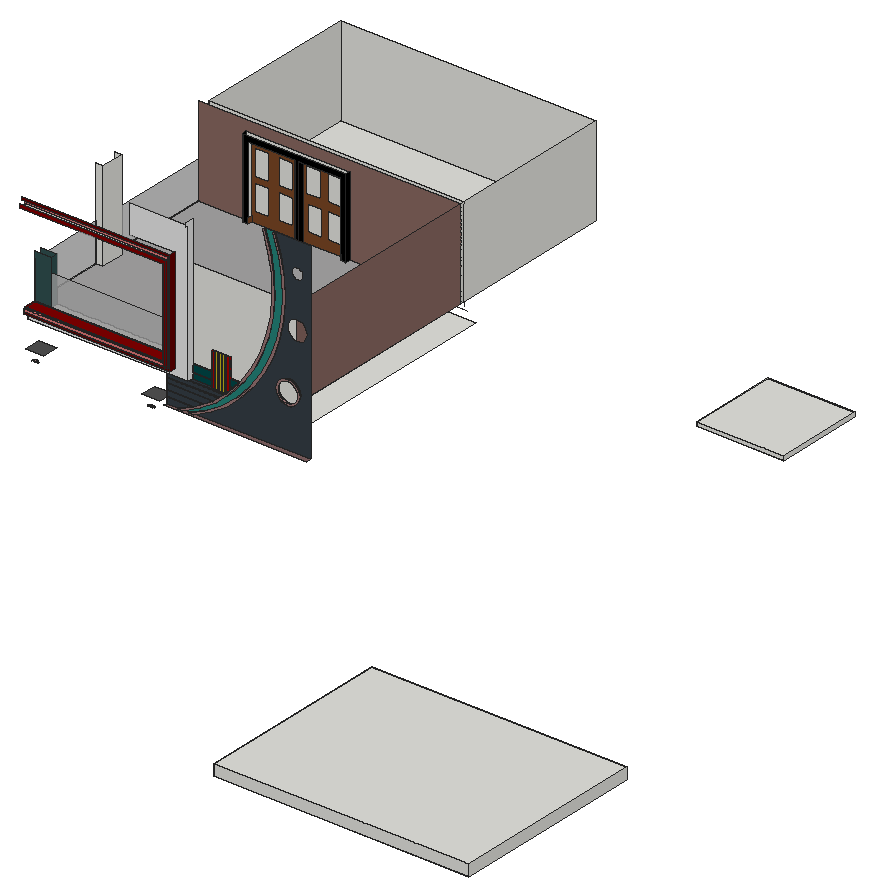
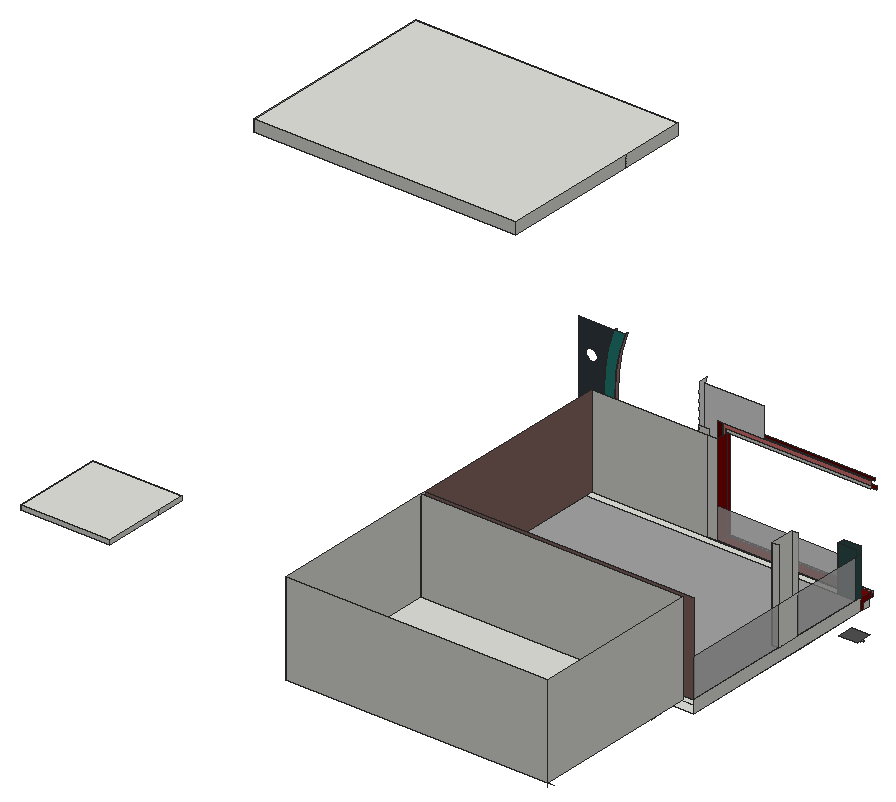
# SketchUp Ruby script. Lengths in inches.
U = 1.inch
M = Sketchup.active_model
def pt(a) = Geom::Point3d.new(a.map { |v| v * U })
def face(e, loops, mat)
  f = e.add_face(loops[0].map { |a| pt(a) })
  loops[1..].each { |l| e.add_face(l.map { |a| pt(a) }).erase! }
  f.material = f.back_material = mat if mat
  f
end
# faces: each face lists its corners as indices into pts; further lists are holes
def faces(e, pts, list, mat = nil) = list.each { |f| face(e, (f[0].is_a?(Array) ? f : [f]).map { |l| l.map { |i| pts[i] } }, mat) }
# xy, xz, yz: faces in a plane at the given z, y or x. An outline is a flat list of corners, or four numbers for a rectangle; further outlines are holes
def ring(l) = l.size == 4 ? [[l[0], l[1]], [l[2], l[1]], [l[2], l[3]], [l[0], l[3]]] : l.each_slice(2).to_a
def flat(e, list, mat, &to3) = list.each { |f| face(e, (f[0].is_a?(Array) ? f : [f]).map { |l| ring(l).map { |u, v| to3.(u, v) } }, mat) }
def xy(e, z, list, mat = nil) = flat(e, list, mat) { |x, y| [x, y, z] }
def xz(e, y, list, mat = nil) = flat(e, list, mat) { |x, z| [x, y, z] }
def yz(e, x, list, mat = nil) = flat(e, list, mat) { |y, z| [x, y, z] }
def lines(e, pts, list) = list.each { |a, b| e.add_line(pt(pts[a]), pt(pts[b])) }
# prism: a flat outline (further loops are holes) pulled along v
def prism(e, loops, v, mat = nil)
  f = face(e, loops, mat); d = Geom::Vector3d.new(v.map { |x| x * U })
  f.pushpull(f.normal.samedirection?(d) ? d.length : -d.length)
end
def box(e, o, s, mat = nil) = prism(e, [[o, [o[0] + s[0], o[1], o[2]], [o[0] + s[0], o[1] + s[1], o[2]], [o[0], o[1] + s[1], o[2]]]], [0, 0, s[2]], mat)
def at(x, y, z, deg = 0) = Geom::Transformation.translation(pt([x, y, z])) * Geom::Transformation.rotation(ORIGIN, Z_AXIS, deg.degrees)
def axes(o, x, y, z) = Geom::Transformation.new([*x, 0, *y, 0, *z, 0, *pt(o).to_a, 1])
def part(name) = M.definitions.add(name)
# library, detail: a bought-in or finely detailed component or shape, given as its bounding box
def library(name, o, s) = part(name).tap { |d| box(d.entities, o, s) }
def detail(e, o, s) = box(e.add_group.entities, o, s)
def put(e, d, t, mat = nil) = e.add_instance(d, t).tap { |i| i.material = mat if mat }
def group(e, t, mat = nil) = e.add_group.tap { |g| g.transformation = t; g.material = mat if mat }.entities
root = M.entities
M.materials.add("[0013_LightCoral]").color = [221, 118, 118]
M.materials.add("[0018_Brown]").color = [165, 42, 42]
M.materials.add("[0020_Red]").color = [165, 0, 0]
M.materials.add("[0022_Maroon]").color = [99, 0, 0]
M.materials.add("[0022_Maroon]1").color = [128, 0, 0]
M.materials.add("[0038_Orange]").color = [214, 196, 27]
M.materials.add("[0046_Gold]").color = [255, 215, 0]
M.materials.add("[0048_PaleGoldenrod]").color = [238, 232, 170]
M.materials.add("[0078_DarkSlateGray]").color = [47, 79, 79]
M.materials.add("[0085_Turquoise]").color = [37, 130, 120]
M.materials.add("[0110_LightSlateGray]").color = [53, 61, 68]
M.materials.add("[0119_RosyBrown]").color = [150, 114, 114]
M.materials.add("[0119_RosyBrown]1").color = [124, 95, 95]
M.materials.add("[0119_RosyBrown]2").color = [170, 129, 129]
M.materials.add("[0133_Gray]").color = [128, 128, 128]
M.materials.add("[0135_DarkGray]").color = [81, 81, 81]
M.materials.add("[0137_Black]").color = [0, 0, 0]
M.materials.add("[Color H08]").color = [0, 71, 71]
M.materials.add("[Polished Concrete Old]").color = [229, 229, 229]
M.materials.add("[Stone Vein Gray]").color = [166, 165, 165]
M.materials.add("[Tile Mosaic Multi]").color = [135, 103, 96]
M.materials.add("[Translucent Resin Crush Gray]").color = [184, 184, 184]
M.materials["[Translucent Resin Crush Gray]"].alpha = 0.8
M.materials.add("[Wood Veneer 01]").color = [120, 70, 37]
xy(root,67.2,[[202.92,648.11,209.75,651.11],[217,648.11,223.83,651.11],[186.0625,650.11,202.92,651.11]])
xy(root,67.2,[[186.0625,645.11,377.9375,645.11,377.9375,651.11,223.83,651.11,223.83,648.11,217,648.11,217,651.11,209.75,651.11,209.75,648.11,202.92,648.11,202.92,650.11,186.0625,650.11]],"[0119_RosyBrown]1")
xy(root,74.96,[[186.0625,650.11,217,651.11],[217,650.11,219.42,651.11]],"[0110_LightSlateGray]")
xy(root,75,[[7,639.11,31.33,660.11],[162.58,639.11,186.0625,639.11,186.0625,654.11,186.19,654.11,186.19,660.11,162.58,660.11]],"[0135_DarkGray]")
xy(root,76.56,[[186.0625,650.11,222.84,651.11]],"[0110_LightSlateGray]")
xy(root,76.8,[[81.13,924.36,101.5,927.36],[107.04,924.36,121.875,927.36]],"[Wood Veneer 01]")
xy(root,83,[[186.0625,650.11,233.5,651.11]],"[0110_LightSlateGray]")
xy(root,84,[[60.84,921.36,73.93,927.36],[73.93,921.36,129.08,924.36],[129.08,921.36,144.84,927.36]],"[0137_Black]")
xy(root,84.34,[[186.0625,650.11,235.92,651.11]],"[0110_LightSlateGray]")
xy(root,90,[[54.84,921.36,150.84,927.36]],"[0137_Black]")
xy(root,91.34,[[186.0625,650.11,246.25,651.11]],"[0110_LightSlateGray]")
xy(root,92.59,[[186.0625,650.11,248.65,651.11]],"[0110_LightSlateGray]")
xy(root,98.34,[[186.0625,650.11,255.49,651.11]],"[0110_LightSlateGray]")
xy(root,99.5625,[[186.0625,650.11,256.95,651.11]],"[0110_LightSlateGray]")
xy(root,104.51,[[[894.52,58.625,894.52,191.3125,979.04,191.3125,979.04,121.17,904.91,121.17,904.91,69.01,1001.94,69.01,1001.94,180.92,992.15,180.92,992.15,191.3125,1012.33,191.3125,1012.33,58.625],[904.91,130.17,970.04,180.92]],[[736.35,929.58,736.35,988.81,765.1,988.81,765.1,957.5,739.89,957.5,739.89,934.22,772.9,934.22,772.9,984.17,769.57,984.17,769.57,988.81,776.43,988.81,776.43,929.58],[739.89,961.52,762.04,984.17]]],"[0018_Brown]")
xy(root,105.125,[[186.0625,650.11,263.57,651.11]],"[0110_LightSlateGray]")
xy(root,106.85,[[[693.78,903.42,810.12,1021.37],[696.84,907.43,807.06,1017.35]],[[736.35,929.58,776.43,929.58,776.43,988.81,769.57,988.81,769.57,984.17,772.9,984.17,772.9,934.22,739.89,934.22,739.89,957.5,765.1,957.5,765.1,988.81,736.35,988.81],[739.89,961.52,762.04,984.17]]])
xy(root,106.85,[[[705.94,919.37,797.96,1005.41],[736.35,929.58,776.43,929.58,776.43,988.81,769.57,988.81,769.57,984.17,772.9,984.17,772.9,934.22,739.89,934.22,739.89,957.5,765.1,957.5,765.1,988.81,736.35,988.81]],[739.89,961.52,762.04,984.17]],"[0048_PaleGoldenrod]")
xy(root,108.55,[[252.74,648.11,252.74,649.11,247.97,649.11,247.97,651.11,271.25,651.11,271.25,649.11,266.58,649.11,266.58,648.11,265.61,648.11,265.61,649.11,253.7,649.11,253.7,648.11]],"[0020_Red]")
xy(root,108.55,[[257.51,648.11,259.2,649.11],[261.76,648.11,263.45,649.11]],"[0038_Orange]")
xy(root,108.56,[[221.0625,650.11,247.97,651.11]],"[Color H08]")
xy(root,109.19,[[[696.84,907.43,807.06,1017.35],[705.94,919.37,797.96,1005.41]]],"[0046_Gold]")
xy(root,109.5,[[186.0625,654.03,207.9375,654.11],[7,654.11,7,756.09,29,756.09,29,787.78,7,787.78,7,927.36,377.9375,927.36,377.9375,654.11],[7,756.09,29,787.78]])
xy(root,109.5,[[7,642.11,221.0625,651.11],[7,651.11,186.0625,654.03]],"[Polished Concrete Old]")
xy(root,110.51,[[[769.37,0,1111.37,264.25],[778.37,9,1102.37,255.25]],[[894.52,58.625,1012.33,58.625,1012.33,191.3125,992.15,191.3125,992.15,180.92,1001.94,180.92,1001.94,69.01,904.91,69.01,904.91,121.17,979.04,121.17,979.04,191.3125,894.52,191.3125],[904.91,130.17,970.04,180.92]]])
xy(root,110.51,[[[805.11,35.75,1075.62,228.5],[894.52,58.625,1012.33,58.625,1012.33,191.3125,992.15,191.3125,992.15,180.92,1001.94,180.92,1001.94,69.01,904.91,69.01,904.91,121.17,979.04,121.17,979.04,191.3125,894.52,191.3125]],[904.91,130.17,970.04,180.92]],"[0048_PaleGoldenrod]")
xy(root,112.7,[[693.78,903.42,810.12,1021.37]])
xy(root,116.06,[[221.0625,650.11,247.97,651.11],[271.25,650.11,274.58,651.11]],"[Color H08]")
xy(root,116.51,[[[778.37,9,1102.37,255.25],[805.11,35.75,1075.62,228.5]]],"[0046_Gold]")
xy(root,117.62,[[221.0625,650.11,247.97,651.11],[271.25,650.11,276.01,651.11]],"[Color H08]")
xy(root,118.06,[[7,642.11,203.6875,651.11]])
xy(root,118.06,[[7,634.61,203.6875,637.61],[7,637.61,203.6875,642.11]],"[0022_Maroon]")
xy(root,120.84,[[7,634.61,200.08,637.61]],"[0022_Maroon]")
xy(root,121.33,[[7,634.61,197.0625,637.61]],"[0013_LightCoral]")
xy(root,124.99,[[7,634.61,193.58,637.61]],"[0013_LightCoral]")
xy(root,124.99,[[7,637.61,194.39,654.03]],"[0022_Maroon]1")
xy(root,125.51,[[769.37,0,1111.37,264.25],[29.57,654.11,358,663.11],[7,756.4375,16,787.78],[16,933.36,358,1154.11]])
xy(root,125.51,[[7,663.11,358,663.11,358,927.36,209.75,927.36,209.75,921.36,202.43,921.36,202.43,927.36,146.28,927.36,146.28,921.36,140.28,921.36,140.28,927.36,78.125,927.36,78.125,921.36,70.81,921.36,70.81,927.36,7,927.36,7,787.78,16,787.78,16,756.4375,7,756.4375]],"[Stone Vein Gray]")
xz(root,0,[[769.37,110.51,1111.37,125.51]])
xz(root,9,[[778.37,110.51,1102.37,116.51]])
xz(root,35.75,[[805.11,110.51,1075.62,116.51]],"[0048_PaleGoldenrod]")
xz(root,58.625,[[894.52,104.51,1012.33,110.51]],"[0018_Brown]")
xz(root,69.01,[[904.91,104.51,1001.94,110.51]],"[0018_Brown]")
xz(root,121.17,[[904.91,104.51,979.04,110.51]],"[0018_Brown]")
xz(root,130.17,[[904.91,104.51,970.04,110.51]],"[0018_Brown]")
xz(root,180.92,[[904.91,104.51,970.04,110.51],[992.15,104.51,1001.94,110.51]],"[0018_Brown]")
xz(root,191.3125,[[894.52,104.51,979.04,110.51],[992.15,104.51,1012.33,110.51]],"[0018_Brown]")
xz(root,228.5,[[805.11,110.51,1075.62,116.51]],"[0048_PaleGoldenrod]")
xz(root,255.25,[[778.37,110.51,1102.37,116.51]])
xz(root,264.25,[[769.37,110.51,1111.37,125.51]])
xz(root,634.61,[[7,121.33,193.58,124.99]],"[0013_LightCoral]")
xz(root,634.61,[[7,118.06,203.6875,118.06,203.6875,258.06,4.6875,258.06,4.6875,254.68,200.08,254.68,200.08,120.84,7,120.84]],"[0022_Maroon]")
xz(root,634.61,[[193.58,121.33,197.0625,121.33,197.0625,248.7,2.625,248.7,2.625,244.39,193.58,244.39]],"[0022_Maroon]1")
xz(root,637.61,[[7,121.33,7,124.99,194.39,124.99,194.39,245.51,7.28,245.51,7.28,248.7,197.0625,248.7,197.0625,121.33],[193.58,124.99,194.39,244.39]])
xz(root,637.61,[[7,120.84,200.08,120.84,200.08,254.68,7,254.68,7,248.7,197.0625,248.7,197.0625,121.33,7,121.33]],"[0013_LightCoral]")
xz(root,642.11,[[7,109.5,221.0625,109.5,221.0625,296.25,143.09,296.25,143.09,258.06,203.6875,258.06,203.6875,118.06,7,118.06]],"[Polished Concrete Old]")
xz(root,648.11,[[252.74,108.55,253.7,152.96],[257.51,108.55,259.2,152.96],[261.76,108.55,263.45,152.96],[265.61,108.55,266.58,152.96]],"[0038_Orange]")
xz(root,648.11,[[202.92,67.2,209.75,67.2,232.66,78.67,253.91,92.99,273.14,109.9,290.05,129.14,304.36,150.39,315.82,173.3,324.26,197.49,329.52,222.56,331.53,248.09,330.25,273.68,325.7,298.89,317.96,323.31,316.26,323.31,323.87,298.58,328.2,273.08,329.19,247.23,326.83,221.48,321.14,196.24,312.23,171.96,300.25,149.04,285.39,127.86,267.92,108.79,248.125,92.14,226.33,78.2],[217,67.2,223.83,67.2,246.74,78.67,267.98,92.99,287.22,109.9,304.13,129.14,318.4375,150.39,329.9,173.3,338.33,197.49,343.6,222.56,345.61,248.09,344.33,273.68,339.78,298.89,332.04,323.31,330.34,323.31,337.94,298.58,342.28,273.08,343.27,247.23,340.9,221.48,335.22,196.24,326.31,171.96,314.33,149.04,299.47,127.86,282,108.79,262.2,92.14,240.41,78.2],[[350.08,122.87,354.18,123.41,357.99,124.99,361.27,127.5,363.78,130.78,365.36,134.59,365.9,138.68,365.36,142.77,363.78,146.59,361.27,149.86,357.99,152.375,354.18,153.96,350.08,154.49,345.99,153.96,342.18,152.375,338.9,149.86,336.39,146.59,334.8125,142.77,334.27,138.68,334.8125,134.59,336.39,130.78,338.9,127.5,342.18,124.99,345.99,123.41],[350.08,125.13,346.58,125.6,343.3125,126.95,340.5,129.1,338.35,131.91,337,135.18,336.54,138.68,337,142.1875,338.35,145.46,340.5,148.26,343.3125,150.41,346.58,151.77,350.08,152.23,353.59,151.77,356.86,150.41,359.66,148.26,361.82,145.46,363.17,142.1875,363.63,138.68,363.17,135.18,361.82,131.91,359.66,129.1,356.86,126.95,353.59,125.6]]],"[0119_RosyBrown]")
xz(root,649.11,[[257.51,108.55,259.2,152.96],[261.76,108.55,263.45,152.96]])
xz(root,649.11,[[247.97,108.55,252.74,152.96],[253.7,108.55,257.51,152.96],[263.45,108.55,265.61,152.96],[266.58,108.55,271.25,152.96]],"[0020_Red]")
xz(root,649.11,[[259.2,108.55,261.76,152.96]],"[0133_Gray]")
xz(root,650.11,[[186.0625,67.2,202.92,67.2,217,73.82,219.42,74.96,186.0625,74.96],[186.0625,76.56,222.84,76.56,226.33,78.2,233.5,82.79,233.5,83,186.0625,83],[186.0625,84.34,235.92,84.34,246.25,90.94,246.25,91.34,186.0625,91.34],[186.0625,92.59,248.65,92.59,255.49,98.34,186.0625,98.34],[186.0625,99.5625,256.95,99.5625,263.57,105.125,186.0625,105.125]],"[0110_LightSlateGray]")
xz(root,650.11,[[221.0625,108.56,247.97,116.06],[271.25,112.42,274.58,116.06,271.25,116.06],[221.0625,117.62,247.97,126.49],[271.25,117.62,276.01,117.62,284.14,126.49,271.25,126.49]],"[Color H08]")
xz(root,651.11,[[202.92,67.2,209.75,67.2,217,70.83,217,73.82],[217,70.83,228.43,76.56,222.84,76.56,219.42,74.96,217,73.82],[186.0625,76.56,186.0625,83,233.5,83,233.5,82.79,226.33,78.2,222.84,76.56],[222.84,76.56,228.43,76.56,232.66,78.67,233.5,79.24,233.5,82.79,226.33,78.2],[233.5,79.24,241.06,84.34,235.92,84.34,233.5,82.79],
  [186.0625,84.34,186.0625,91.34,246.25,91.34,246.25,90.94,235.92,84.34],[235.92,84.34,241.06,84.34,246.25,87.83,246.25,90.94],[246.25,87.83,253.3125,92.59,248.65,92.59,248.125,92.14,246.25,90.94],[186.0625,92.59,186.0625,98.34,255.49,98.34,248.65,92.59],[248.65,92.59,253.3125,92.59,253.91,92.99,259.99,98.34,255.49,98.34],
  [255.49,98.34,259.99,98.34,261.39,99.5625,256.95,99.5625],[186.0625,99.5625,186.0625,105.125,263.57,105.125,256.95,99.5625],[256.95,99.5625,261.39,99.5625,267.5,104.9375,267.5,105.125,263.57,105.125],[267.5,104.9375,271.61,108.56,271.25,108.56,271.25,108.55,267.64,108.55,263.57,105.125,267.5,105.125],[247.97,108.55,247.97,108.56,267.65,108.56,267.64,108.55],
  [267.64,108.55,267.71,108.55,267.71,108.56,267.65,108.56],[267.71,108.55,271.25,108.56],[221.0625,108.56,247.97,116.06],[247.97,108.56,247.97,108.61,267.71,108.61,267.65,108.56],[267.65,108.56,267.71,108.61,267.71,108.56],
  [267.71,108.56,271.25,108.61],[271.25,108.56,271.61,108.56,273.14,109.9,278.55,116.06,274.58,116.06,271.25,112.42],[247.97,108.61,247.97,112.42,271.25,112.42,267.92,108.79,267.71,108.61],[267.71,108.61,271.25,108.61,271.25,112.42,267.92,108.79],[207.9375,109.5,221.0625,251.36],
  [247.97,112.42,271.25,152.96],[271.25,112.42,271.25,116.06,274.58,116.06],[274.58,116.06,278.55,116.06,279.92,117.62,276.01,117.62],[221.0625,117.62,247.97,126.49],[271.25,117.62,271.25,126.49,284.14,126.49,276.01,117.62],
  [276.01,117.62,279.92,117.62,286.25,124.81,286.25,126.49,284.14,126.49],[286.25,124.81,289.23,128.2,285.64,128.2,285.39,127.86,284.14,126.49,286.25,126.49],[350.08,125.13,353.59,125.6,356.86,126.95,359.66,129.1,361.82,131.91,363.17,135.18,363.63,138.68,363.17,142.1875,361.82,145.46,359.66,148.26,356.86,150.41,353.59,151.77,350.08,152.23,346.58,151.77,343.3125,150.41,340.5,148.26,338.35,145.46,337,142.1875,336.54,138.68,337,135.18,338.35,131.91,340.5,129.1,343.3125,126.95,346.58,125.6]])
xz(root,651.11,[[209.75,67.2,217,67.2,240.41,78.2,262.2,92.14,282,108.79,299.47,127.86,314.33,149.04,326.31,171.96,335.22,196.24,340.9,221.48,343.27,247.23,342.28,273.08,337.94,298.58,330.34,323.31,317.96,323.31,319.04,319.9,322.13,310.14,324.59,302.39,325.11,300.74,325.7,298.89,327.19,290.61,327.54,288.67,329.16,279.73,329.47,278.01,330.25,273.68,330.41,270.44,330.5,268.56,330.96,259.56,331.03,258.11,331.53,248.09,331.5,247.73,331.29,245.03,330.49,234.84,330.31,232.54,329.52,222.56,329.49,222.41,329.12,220.65,326.59,208.59,325.82,204.94,324.26,197.49,323.04,194,322.05,191.16,318.32,180.47,317.53,178.2,315.82,173.3,312.62,166.89,311.48,164.61,305.64,152.96,304.36,150.39,303.45,149.04,297.18,139.72,294.98,136.45,290.05,129.14,289.23,128.2,286.25,124.81,279.92,117.62,278.55,116.06,273.14,109.9,271.61,108.56,267.5,104.9375,261.39,99.5625,259.99,98.34,253.91,92.99,253.3125,92.59,246.25,87.83,241.06,84.34,233.5,79.24,232.66,78.67,228.43,76.56,217,70.83]],"[0085_Turquoise]")
xz(root,651.11,[[[223.83,67.2,377.9375,67.2,377.9375,323.31,332.04,323.31,339.78,298.89,344.33,273.68,345.61,248.09,343.6,222.56,338.33,197.49,329.9,173.3,318.4375,150.39,304.13,129.14,287.22,109.9,267.98,92.99,246.74,78.67],[350.08,122.87,345.99,123.41,342.18,124.99,338.9,127.5,336.39,130.78,334.8125,134.59,334.27,138.68,334.8125,142.77,336.39,146.59,338.9,149.86,342.18,152.375,345.99,153.96,350.08,154.49,354.18,153.96,357.99,152.375,361.27,149.86,363.78,146.59,365.36,142.77,365.9,138.68,365.36,134.59,363.78,130.78,361.27,127.5,357.99,124.99,354.18,123.41],[360.63,201.66,357.15,202.12,353.91,203.46,351.12,205.6,348.98,208.39,347.64,211.63,347.18,215.11,347.64,218.6,348.98,221.84,351.12,224.63,353.91,226.76,357.15,228.11,360.63,228.57,364.12,228.11,367.36,226.76,370.15,224.63,372.29,221.84,373.63,218.6,374.09,215.11,373.63,211.63,372.29,208.39,370.15,205.6,367.36,203.46,364.12,202.12],[360.63,275.86,358.68,276.11,356.85,276.87,355.29,278.07,354.09,279.64,353.33,281.46,353.07,283.42,353.33,285.375,354.09,287.2,355.29,288.77,356.85,289.97,358.68,290.72,360.63,290.98,362.59,290.72,364.42,289.97,365.98,288.77,367.18,287.2,367.94,285.375,368.2,283.42,367.94,281.46,367.18,279.64,365.98,278.07,364.42,276.87,362.59,276.11]],[186.0625,74.96,219.42,74.96,222.84,76.56,186.0625,76.56],[233.5,82.79,235.92,84.34,186.0625,84.34,186.0625,83,233.5,83],[246.25,90.94,248.125,92.14,248.65,92.59,186.0625,92.59,186.0625,91.34,246.25,91.34],[186.0625,98.34,255.49,98.34,256.95,99.5625,186.0625,99.5625],
  [186.0625,105.125,263.57,105.125,267.64,108.55,247.97,108.55,247.97,108.56,221.0625,108.56,221.0625,109.5,186.0625,109.5]],"[0110_LightSlateGray]")
xz(root,651.11,[[221.0625,116.06,247.97,117.62],[271.25,116.06,274.58,116.06,276.01,117.62,271.25,117.62]],"[Color H08]")
xz(root,654.03,[[7,109.5,7,124.99,194.39,124.99,194.39,245.51,207.9375,245.51,207.9375,109.5]])
xz(root,654.11,[[207.9375,125.51,358,245.51]])
xz(root,654.11,[[7,109.5,207.9375,109.5,207.9375,125.51,29.57,125.51,29.57,185.51,7,185.51]],"[0078_DarkSlateGray]")
xz(root,663.11,[[7,125.51,29.57,185.51]],"[0078_DarkSlateGray]")
xz(root,756.4375,[[7,125.51,16,245.51]])
xz(root,787.78,[[7,125.51,16,245.51]])
xz(root,903.42,[[693.78,106.85,810.12,112.7]])
xz(root,907.43,[[696.84,106.85,807.06,109.19]])
xz(root,919.37,[[705.94,106.85,797.96,109.19]],"[0048_PaleGoldenrod]")
xz(root,921.36,[[70.81,125.51,78.125,125.51,78.125,224.07,140.28,224.07,140.28,125.51,146.28,125.51,146.28,224.07,202.43,224.07,202.43,125.51,209.75,125.51,209.75,231.39,70.81,231.39]],"[0137_Black]")
xz(root,927.36,[[7,125.51,70.81,125.51,70.81,231.39,209.75,231.39,209.75,125.51,358,125.51,358,245.51,7,245.51]],"[Tile Mosaic Multi]")
xz(root,927.36,[[[78.125,125.51,140.28,224.07],[82.37,181.25,101.18,215.75],[114.12,181.25,132.93,215.75],[114.12,139.3125,132.93,173.8125],[82.93,139.3125,101.74,173.8125]],[[146.28,125.51,202.43,224.07],[179.93,184.8125,198.74,219.3125],[151.49,184.8125,170.3,219.3125],[153.68,139.3125,172.49,173.8125],[179.93,139.3125,198.74,173.8125]]],"[Wood Veneer 01]")
xz(root,929.58,[[736.35,104.51,776.43,106.85]],"[0018_Brown]")
xz(root,933.36,[[16,125.51,358,245.51]])
xz(root,934.22,[[739.89,104.51,772.9,106.85]],"[0018_Brown]")
xz(root,957.5,[[739.89,104.51,765.1,106.85]],"[0018_Brown]")
xz(root,961.52,[[739.89,104.51,762.04,106.85]],"[0018_Brown]")
xz(root,984.17,[[739.89,104.51,762.04,106.85],[769.57,104.51,772.9,106.85]],"[0018_Brown]")
xz(root,988.81,[[736.35,104.51,765.1,106.85],[769.57,104.51,776.43,106.85]],"[0018_Brown]")
xz(root,1005.41,[[705.94,106.85,797.96,109.19]],"[0048_PaleGoldenrod]")
xz(root,1017.35,[[696.84,106.85,807.06,109.19]])
xz(root,1021.37,[[693.78,106.85,810.12,112.7]])
xz(root,1154.11,[[16,125.51,358,245.51]])
yz(root,7,[[642.11,109.5,651.11,118.06],[654.11,109.5,927.36,125.51],[756.4375,125.51,787.78,176]])
yz(root,7,[[634.61,121.33,637.61,124.99]],"[0013_LightCoral]")
yz(root,7,[[634.61,118.06,637.61,120.84]],"[0022_Maroon]")
yz(root,7,[[651.11,109.5,651.11,118.06,637.61,118.06,637.61,124.99,654.03,124.99,654.03,109.5]],"[0022_Maroon]1")
yz(root,7,[[654.11,125.51,663.11,176]],"[0078_DarkSlateGray]")
yz(root,7,[[663.11,125.51,756.4375,176],[787.78,125.51,927.36,176]],"[Translucent Resin Crush Gray]")
yz(root,16,[[756.4375,125.51,787.78,245.51],[933.36,125.51,1154.11,245.51]])
yz(root,29.57,[[654.11,125.51,663.11,185.51]],"[0078_DarkSlateGray]")
yz(root,70.81,[[921.36,125.51,927.36,231.39]],"[0137_Black]")
yz(root,78.125,[[921.36,125.51,927.36,132.83]],"[Wood Veneer 01]")
yz(root,140.28,[[921.36,125.51,927.36,224.07]],"[0137_Black]")
yz(root,146.28,[[921.36,125.51,927.36,224.07]],"[0137_Black]")
yz(root,186.0625,[[650.11,67.2,651.11,74.96]])
yz(root,186.0625,[[651.11,75,654.11,109.5],[650.11,76.56,651.11,83],[650.11,84.34,651.11,91.34],[650.11,92.59,651.11,98.34],[650.11,99.5625,651.11,105.125]],"[0110_LightSlateGray]")
yz(root,193.58,[[634.61,124.99,637.61,244.39]],"[0022_Maroon]1")
yz(root,194.39,[[637.61,124.99,654.03,245.51]],"[0022_Maroon]1")
yz(root,197.0625,[[634.61,121.33,637.61,248.7]],"[0022_Maroon]1")
yz(root,200.08,[[634.61,120.84,637.61,254.68]],"[0022_Maroon]")
yz(root,202.43,[[921.36,125.51,927.36,132.83]],"[Wood Veneer 01]")
yz(root,203.6875,[[634.61,118.06,642.11,258.06]],"[0022_Maroon]")
yz(root,209.75,[[921.36,125.51,927.36,231.39]],"[0137_Black]")
yz(root,221.0625,[[650.11,108.56,651.11,109.5],[650.11,109.5,651.11,116.06],[650.11,117.62,651.11,126.49]])
yz(root,221.0625,[[642.11,109.5,650.11,109.5,650.11,116.06,651.11,116.06,651.11,117.62,650.11,117.62,650.11,126.49,651.11,126.49,651.11,128.2,650.11,128.2,650.11,136.45,651.11,136.45,651.11,139.72,650.11,139.72,650.11,149.04,651.11,149.04,651.11,152.96,650.11,152.96,650.11,164.61,651.11,164.61,651.11,166.89,650.11,166.89,650.11,178.2,651.11,178.2,651.11,180.47,650.11,180.47,650.11,191.16,651.11,191.16,651.11,194,650.11,194,650.11,204.94,651.11,204.94,651.11,208.59,650.11,208.59,650.11,220.65,651.11,220.65,651.11,222.41,650.11,222.41,650.11,232.54,651.11,232.54,651.11,234.84,650.11,234.84,650.11,245.03,651.11,245.03,651.11,247.73,650.11,247.73,650.11,258.11,651.11,258.11,651.11,259.56,650.11,259.56,650.11,268.56,651.11,268.56,651.11,270.44,650.11,270.44,650.11,278.01,651.11,278.01,651.11,279.73,650.11,279.73,650.11,288.67,651.11,288.67,651.11,290.61,650.11,290.61,650.11,300.74,638.11,300.74,638.11,299.9,639.11,299.9,639.11,296.25,642.11,296.25]],"[Polished Concrete Old]")
yz(root,233.5,[[650.11,82.79,651.11,83]],"[0110_LightSlateGray]")
yz(root,246.25,[[650.11,90.94,651.11,91.34]],"[0110_LightSlateGray]")
yz(root,247.97,[[649.11,108.55,649.11,108.61,650.11,108.61,650.11,108.56,651.11,108.56,651.11,108.55],[650.11,108.56,651.11,108.61],[650.11,108.61,651.11,112.42],[650.11,112.42,651.11,116.06],[650.11,117.62,651.11,126.49]])
yz(root,247.97,[[649.11,108.61,649.11,152.96,651.11,152.96,651.11,149.04,650.11,149.04,650.11,139.72,651.11,139.72,651.11,136.45,650.11,136.45,650.11,128.2,651.11,128.2,651.11,126.49,650.11,126.49,650.11,117.62,651.11,117.62,651.11,116.06,650.11,116.06,650.11,108.61]],"[0020_Red]")
yz(root,252.74,[[648.11,108.55,649.11,152.96]],"[0038_Orange]")
yz(root,253.7,[[648.11,108.55,649.11,152.96]],"[0038_Orange]")
yz(root,257.51,[[648.11,108.55,649.11,152.96]],"[0038_Orange]")
yz(root,259.2,[[648.11,108.55,649.11,152.96]],"[0038_Orange]")
yz(root,261.76,[[648.11,108.55,649.11,152.96]],"[0038_Orange]")
yz(root,263.45,[[648.11,108.55,649.11,152.96]],"[0038_Orange]")
yz(root,265.61,[[648.11,108.55,649.11,152.96]],"[0038_Orange]")
yz(root,266.58,[[648.11,108.55,649.11,152.96]],"[0038_Orange]")
yz(root,271.25,[[649.11,108.55,651.11,108.61],[649.11,108.61,651.11,112.42],[650.11,112.42,651.11,116.06],[650.11,117.62,651.11,126.49]])
yz(root,271.25,[[649.11,112.42,650.11,112.42,650.11,116.06,651.11,116.06,651.11,117.62,650.11,117.62,650.11,126.49,651.11,126.49,651.11,128.2,650.11,128.2,650.11,136.45,651.11,136.45,651.11,139.72,650.11,139.72,650.11,149.04,651.11,149.04,651.11,152.96,649.11,152.96]],"[0020_Red]")
yz(root,358,[[927.36,125.51,933.36,245.51],[933.36,125.51,1154.11,245.51]])
yz(root,358,[[654.11,125.51,927.36,245.51]],"[Tile Mosaic Multi]")
yz(root,693.78,[[903.42,106.85,941.31,112.7],[941.31,106.85,1021.37,112.7]])
yz(root,696.84,[[907.43,106.85,941.31,109.19],[941.31,106.85,1017.35,109.19]])
yz(root,705.94,[[919.37,106.85,941.31,109.19],[941.31,106.85,1005.41,109.19]])
yz(root,736.35,[[929.58,104.51,988.81,106.85]],"[0018_Brown]")
yz(root,739.89,[[934.22,104.51,957.5,106.85],[961.52,104.51,984.17,106.85]],"[0018_Brown]")
yz(root,762.04,[[961.52,104.51,984.17,106.85]],"[0018_Brown]")
yz(root,765.1,[[957.5,104.51,988.81,106.85]],"[0018_Brown]")
yz(root,769.37,[[0,110.51,84.91,125.51],[84.91,110.51,264.25,125.51]])
yz(root,769.57,[[984.17,104.51,988.81,106.85]],"[0018_Brown]")
yz(root,772.9,[[934.22,104.51,984.17,106.85]],"[0018_Brown]")
yz(root,776.43,[[929.58,104.51,988.81,106.85]],"[0018_Brown]")
yz(root,778.37,[[9,110.51,84.91,116.51],[84.91,110.51,255.25,116.51]])
yz(root,797.96,[[919.37,106.85,1005.41,109.19]])
yz(root,805.11,[[35.75,110.51,84.91,116.51],[84.91,110.51,228.5,116.51]])
yz(root,807.06,[[907.43,106.85,1017.35,109.19]])
yz(root,810.12,[[903.42,106.85,1021.37,112.7]])
yz(root,894.52,[[58.625,104.51,191.3125,110.51]],"[0018_Brown]")
yz(root,904.91,[[69.01,104.51,121.17,110.51],[130.17,104.51,180.92,110.51]],"[0018_Brown]")
yz(root,970.04,[[130.17,104.51,180.92,110.51]],"[0018_Brown]")
yz(root,979.04,[[121.17,104.51,191.3125,110.51]],"[0018_Brown]")
yz(root,992.15,[[180.92,104.51,191.3125,110.51]],"[0018_Brown]")
yz(root,1001.94,[[69.01,104.51,180.92,110.51]],"[0018_Brown]")
yz(root,1012.33,[[58.625,104.51,191.3125,110.51]],"[0018_Brown]")
yz(root,1075.62,[[35.75,110.51,228.5,116.51]])
yz(root,1102.37,[[9,110.51,255.25,116.51]])
yz(root,1111.37,[[0,110.51,264.25,125.51]])
p = [[19.87,641.11,64.46],[19.87,638.11,64.46],[18.01,638.11,64.21],[18.01,641.11,64.21],[21.73,641.11,64.21],[21.73,638.11,64.21],
  [171.7,639.11,64.95],[170.25,639.11,64.24],[170.25,638.11,64.24],[171.7,638.11,64.95],[173.4,641.11,64.6],[173.4,638.11,64.6],
  [171.98,638.11,64.21],[171.98,641.11,64.21],[177.75,641.11,64.21],[177.75,638.11,64.21],[176.33,638.11,64.6],[176.33,641.11,64.6],
  [179.49,639.11,64.24],[178.04,639.11,64.95],[178.04,638.11,64.95],[179.49,638.11,64.24],[17.78,639.11,65.07],[15.83,639.11,64.26],
  [15.83,638.11,64.26],[17.78,638.11,65.07],[23.9,639.11,64.26],[21.96,639.11,65.07],[21.96,638.11,65.07],[23.9,638.11,64.26],
  [174.87,641.11,64.74],[174.87,638.11,64.74],[173.26,639.11,65.39],[173.26,638.11,65.39],[176.48,639.11,65.39],[176.48,638.11,65.39],
  [19.87,639.11,65.35],[19.87,638.11,65.35],[174.87,639.11,65.54],[174.87,638.11,65.54],[222.84,651.11,76.56],[219.42,651.11,74.96],
  [219.42,650.11,74.96],[217,650.11,73.82],[202.92,650.11,67.2],[202.92,648.11,67.2],[226.33,648.11,78.2],[226.33,650.11,78.2],
  [222.84,650.11,76.56],[209.75,651.11,67.2],[217,651.11,70.83],[228.43,651.11,76.56],[232.66,651.11,78.67],[232.66,648.11,78.67],
  [209.75,648.11,67.2],[240.41,651.11,78.2],[217,651.11,67.2],[217,648.11,67.2],[240.41,648.11,78.2],[223.83,651.11,67.2],
  [246.74,651.11,78.67],[246.74,648.11,78.67],[223.83,648.11,67.2],[217,651.11,73.82],[202.92,651.11,67.2],[226.33,651.11,78.2],
  [235.92,651.11,84.34],[233.5,651.11,82.79],[233.5,650.11,82.79],[248.125,648.11,92.14],[248.125,651.11,92.14],[246.25,651.11,90.94],
  [246.25,650.11,90.94],[235.92,650.11,84.34],[262.2,651.11,92.14],[262.2,648.11,92.14],[233.5,651.11,79.24],[241.06,651.11,84.34],
  [246.25,651.11,87.83],[253.3125,651.11,92.59],[253.91,651.11,92.99],[253.91,648.11,92.99],[267.98,651.11,92.99],[267.98,648.11,92.99],
  [248.65,651.11,92.59],[267.92,648.11,108.79],[267.92,651.11,108.79],[267.71,651.11,108.61],[267.65,651.11,108.56],[267.64,651.11,108.55],
  [263.57,651.11,105.125],[263.57,650.11,105.125],[256.95,650.11,99.5625],[256.95,651.11,99.5625],[255.49,651.11,98.34],[255.49,650.11,98.34],
  [248.65,650.11,92.59],[282,651.11,108.79],[282,648.11,108.79],[259.99,651.11,98.34],[261.39,651.11,99.5625],[267.5,651.11,104.9375],
  [271.61,651.11,108.56],[273.14,651.11,109.9],[273.14,648.11,109.9],[287.22,651.11,109.9],[287.22,648.11,109.9],[271.25,651.11,112.42],
  [285.39,648.11,127.86],[285.39,651.11,127.86],[284.14,651.11,126.49],[284.14,650.11,126.49],[276.01,650.11,117.62],[276.01,651.11,117.62],
  [274.58,651.11,116.06],[274.58,650.11,116.06],[271.25,650.11,112.42],[299.47,651.11,127.86],[299.47,648.11,127.86],[278.55,651.11,116.06],
  [279.92,651.11,117.62],[286.25,651.11,124.81],[289.23,651.11,128.2],[290.05,651.11,129.14],[290.05,648.11,129.14],[304.13,651.11,129.14],
  [304.13,648.11,129.14],[345.99,651.11,123.41],[350.08,651.11,122.87],[350.08,648.11,122.87],[345.99,648.11,123.41],[354.18,651.11,123.41],
  [354.18,648.11,123.41],[342.18,651.11,124.99],[342.18,648.11,124.99],[357.99,651.11,124.99],[357.99,648.11,124.99],[338.9,651.11,127.5],
  [338.9,648.11,127.5],[361.27,651.11,127.5],[361.27,648.11,127.5],[350.08,651.11,125.13],[346.58,651.11,125.6],[346.58,648.11,125.6],
  [350.08,648.11,125.13],[353.59,651.11,125.6],[353.59,648.11,125.6],[194.39,654.03,125.51],[29.57,654.11,125.51],[29.57,654.11,166.57],
  [194.39,654.03,166.57],[343.3125,651.11,126.95],[343.3125,648.11,126.95],[356.86,651.11,126.95],[356.86,648.11,126.95],[7,927.36,120],
  [367,927.36,120],[358,933.36,120],[358,933.36,125.51],[16,1154.11,120],[16,1154.11,125.51],[7,1154.11,125.51],
  [358,654.11,125.51],[358,651.11,125.51]]
faces(root,p,[[0,1,2,3],[4,5,1,0],[6,7,8,9],[10,11,12,13],[14,15,16,17],[18,19,20,21],[22,23,24,25],[26,27,28,29],
  [30,31,11,10],[17,16,31,30],[32,6,9,33],[19,34,35,20],[36,22,25,37],[27,36,37,28],[38,32,33,39],[34,38,39,35]],"[0119_RosyBrown]2")
faces(root,p,[[40,41,42,43,44,45,46,47,48],[49,50,51,52,53,54],[55,56,57,58],[59,60,61,62],[66,67,68,47,46,69,70,71,72,73],[74,55,58,75],[52,76,77,78,79,80,81,53],[60,82,83,61],
  [84,70,69,85,86,87,88,89,90,91,92,93,94,95,96],[97,74,75,98],[80,99,100,101,102,103,104,81],[82,105,106,83],[107,86,85,108,109,110,111,112,113,114,115,116],[117,97,98,118],[103,119,120,121,122,123,124,104],[105,125,126,106],
  [127,128,129,130],[128,131,132,129],[133,127,130,134],[131,135,136,132],[137,133,134,138],[135,139,140,136],[141,142,143,144],[145,141,144,146],
  [142,151,152,143],[153,145,146,154]],"[0119_RosyBrown]")
faces(root,p,[[63,64,44,43],[63,43,42,41],[65,40,48,47],[67,65,47,68],[71,66,73,72],[94,84,96,95],[90,93,92,91],[114,107,116,115],
  [110,113,112,111]])
faces(root,p,[[147,148,149,150]],"[Translucent Resin Crush Gray]")
lines(root,p,[[155,156],[157,158],[159,160],[160,161],[162,163]])
